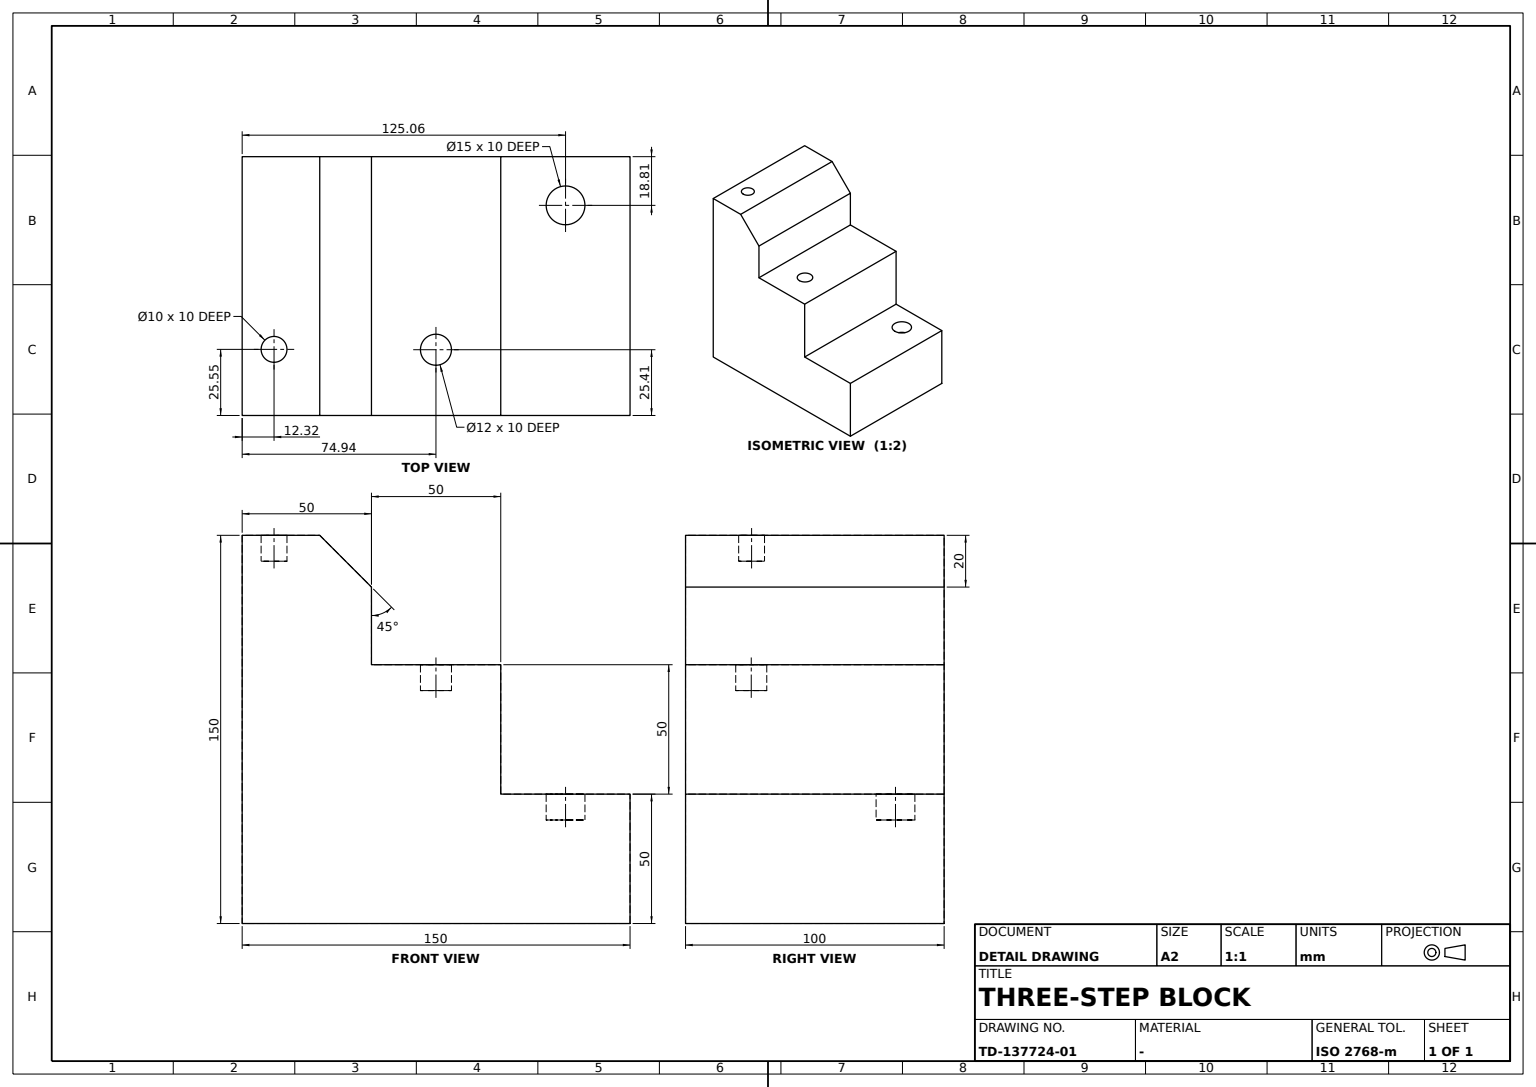
ISO-10303-21;
HEADER;
FILE_DESCRIPTION((''),'2;1');
FILE_NAME('','',(''),(''),'','','');
FILE_SCHEMA(('AUTOMOTIVE_DESIGN'));
ENDSEC;
DATA;
#1=APPLICATION_CONTEXT('');
#2=PRODUCT_CONTEXT('',#1,'mechanical');
#3=PRODUCT('','','',(#2));
#4=PRODUCT_DEFINITION_FORMATION('','',#3);
#5=PRODUCT_DEFINITION_CONTEXT('',#1,'design');
#6=PRODUCT_DEFINITION('','',#4,#5);
#7=PRODUCT_DEFINITION_SHAPE('','',#6);
#8=(LENGTH_UNIT()NAMED_UNIT(*)SI_UNIT(.MILLI.,.METRE.));
#9=(NAMED_UNIT(*)PLANE_ANGLE_UNIT()SI_UNIT($,.RADIAN.));
#10=(NAMED_UNIT(*)SI_UNIT($,.STERADIAN.)SOLID_ANGLE_UNIT());
#11=UNCERTAINTY_MEASURE_WITH_UNIT(LENGTH_MEASURE(0.005),#8,'distance_accuracy_value','');
#12=(GEOMETRIC_REPRESENTATION_CONTEXT(3)GLOBAL_UNCERTAINTY_ASSIGNED_CONTEXT((#11))GLOBAL_UNIT_ASSIGNED_CONTEXT((#8,#9,#10))REPRESENTATION_CONTEXT('',''));
#13=CARTESIAN_POINT('',(-50.,-75.,75.));
#14=VERTEX_POINT('',#13);
#15=CARTESIAN_POINT('',(50.,-75.,75.));
#16=VERTEX_POINT('',#15);
#17=CARTESIAN_POINT('',(0.,-75.,75.));
#18=DIRECTION('',(1.,0.,0.));
#19=VECTOR('',#18,1000.);
#20=LINE('',#17,#19);
#21=EDGE_CURVE('',#14,#16,#20,.T.);
#22=ORIENTED_EDGE('',*,*,#21,.F.);
#23=CARTESIAN_POINT('',(-50.,-75.,-75.));
#24=VERTEX_POINT('',#23);
#25=CARTESIAN_POINT('',(-50.,-75.,0.));
#26=DIRECTION('',(0.,0.,-1.));
#27=VECTOR('',#26,1000.);
#28=LINE('',#25,#27);
#29=EDGE_CURVE('',#14,#24,#28,.T.);
#30=ORIENTED_EDGE('',*,*,#29,.T.);
#31=CARTESIAN_POINT('',(50.,-75.,-75.));
#32=VERTEX_POINT('',#31);
#33=CARTESIAN_POINT('',(0.,-75.,-75.));
#34=LINE('',#33,#19);
#35=EDGE_CURVE('',#24,#32,#34,.T.);
#36=ORIENTED_EDGE('',*,*,#35,.T.);
#37=CARTESIAN_POINT('',(50.,-75.,0.));
#38=LINE('',#37,#27);
#39=EDGE_CURVE('',#16,#32,#38,.T.);
#40=ORIENTED_EDGE('',*,*,#39,.F.);
#41=EDGE_LOOP('',(#22,#30,#36,#40));
#42=FACE_BOUND('',#41,.T.);
#43=DIRECTION('',(0.,-1.,0.));
#44=AXIS2_PLACEMENT_3D('',#17,#43,#26);
#45=PLANE('',#44);
#46=ADVANCED_FACE('',(#42),#45,.T.);
#47=CARTESIAN_POINT('',(-38.687384,50.059444,-35.));
#48=VERTEX_POINT('',#47);
#49=CARTESIAN_POINT('',(-31.187384,50.059444,-35.));
#50=DIRECTION('',(-1.,0.,0.));
#51=AXIS2_PLACEMENT_3D('',#49,#26,#50);
#52=CIRCLE('',#51,7.5);
#53=EDGE_CURVE('',#48,#48,#52,.T.);
#54=ORIENTED_EDGE('',*,*,#53,.T.);
#55=EDGE_LOOP('',(#54));
#56=FACE_BOUND('',#55,.T.);
#57=CARTESIAN_POINT('',(-23.687384,50.059444,-25.));
#58=VERTEX_POINT('',#57);
#59=CARTESIAN_POINT('',(-31.187384,50.059444,-25.));
#60=DIRECTION('',(0.,0.,1.));
#61=AXIS2_PLACEMENT_3D('',#59,#60,#18);
#62=CIRCLE('',#61,7.5);
#63=EDGE_CURVE('',#58,#58,#62,.T.);
#64=ORIENTED_EDGE('',*,*,#63,.T.);
#65=EDGE_LOOP('',(#64));
#66=FACE_BOUND('',#65,.T.);
#67=CARTESIAN_POINT('',(-31.187384,50.059444,-25.1));
#68=AXIS2_PLACEMENT_3D('',#67,#26,#18);
#69=CYLINDRICAL_SURFACE('',#68,7.5);
#70=ADVANCED_FACE('',(#56,#66),#69,.F.);
#71=CARTESIAN_POINT('',(19.454487,-62.675179,65.));
#72=VERTEX_POINT('',#71);
#73=CARTESIAN_POINT('',(24.454487,-62.675179,65.));
#74=AXIS2_PLACEMENT_3D('',#73,#26,#50);
#75=CIRCLE('',#74,5.);
#76=EDGE_CURVE('',#72,#72,#75,.T.);
#77=ORIENTED_EDGE('',*,*,#76,.F.);
#78=EDGE_LOOP('',(#77));
#79=FACE_BOUND('',#78,.T.);
#80=AXIS2_PLACEMENT_3D('',#73,#26,#18);
#81=PLANE('',#80);
#82=ADVANCED_FACE('',(#79),#81,.F.);
#83=ORIENTED_EDGE('',*,*,#53,.F.);
#84=EDGE_LOOP('',(#83));
#85=FACE_BOUND('',#84,.T.);
#86=AXIS2_PLACEMENT_3D('',#49,#26,#18);
#87=PLANE('',#86);
#88=ADVANCED_FACE('',(#85),#87,.F.);
#89=CARTESIAN_POINT('',(-50.,25.,25.));
#90=VERTEX_POINT('',#89);
#91=CARTESIAN_POINT('',(50.,25.,25.));
#92=VERTEX_POINT('',#91);
#93=CARTESIAN_POINT('',(0.,25.,25.));
#94=LINE('',#93,#19);
#95=EDGE_CURVE('',#90,#92,#94,.T.);
#96=ORIENTED_EDGE('',*,*,#95,.F.);
#97=CARTESIAN_POINT('',(-50.,-25.,25.));
#98=VERTEX_POINT('',#97);
#99=CARTESIAN_POINT('',(-50.,0.,25.));
#100=VECTOR('',#43,1000.);
#101=LINE('',#99,#100);
#102=EDGE_CURVE('',#90,#98,#101,.T.);
#103=ORIENTED_EDGE('',*,*,#102,.T.);
#104=CARTESIAN_POINT('',(50.,-25.,25.));
#105=VERTEX_POINT('',#104);
#106=CARTESIAN_POINT('',(0.,-25.,25.));
#107=LINE('',#106,#19);
#108=EDGE_CURVE('',#98,#105,#107,.T.);
#109=ORIENTED_EDGE('',*,*,#108,.T.);
#110=CARTESIAN_POINT('',(50.,0.,25.));
#111=LINE('',#110,#100);
#112=EDGE_CURVE('',#92,#105,#111,.T.);
#113=ORIENTED_EDGE('',*,*,#112,.F.);
#114=EDGE_LOOP('',(#96,#103,#109,#113));
#115=FACE_BOUND('',#114,.T.);
#116=CARTESIAN_POINT('',(30.590931,-0.059691,25.));
#117=VERTEX_POINT('',#116);
#118=CARTESIAN_POINT('',(24.590931,-0.059691,25.));
#119=AXIS2_PLACEMENT_3D('',#118,#60,#18);
#120=CIRCLE('',#119,6.);
#121=EDGE_CURVE('',#117,#117,#120,.T.);
#122=ORIENTED_EDGE('',*,*,#121,.F.);
#123=EDGE_LOOP('',(#122));
#124=FACE_BOUND('',#123,.T.);
#125=AXIS2_PLACEMENT_3D('',#93,#60,#43);
#126=PLANE('',#125);
#127=ADVANCED_FACE('',(#115,#124),#126,.T.);
#128=CARTESIAN_POINT('',(-50.,25.,-25.));
#129=VERTEX_POINT('',#128);
#130=CARTESIAN_POINT('',(-50.,25.,0.));
#131=VECTOR('',#60,1000.);
#132=LINE('',#130,#131);
#133=EDGE_CURVE('',#129,#90,#132,.T.);
#134=ORIENTED_EDGE('',*,*,#133,.T.);
#135=ORIENTED_EDGE('',*,*,#95,.T.);
#136=CARTESIAN_POINT('',(50.,25.,-25.));
#137=VERTEX_POINT('',#136);
#138=CARTESIAN_POINT('',(50.,25.,0.));
#139=LINE('',#138,#131);
#140=EDGE_CURVE('',#137,#92,#139,.T.);
#141=ORIENTED_EDGE('',*,*,#140,.F.);
#142=CARTESIAN_POINT('',(0.,25.,-25.));
#143=LINE('',#142,#19);
#144=EDGE_CURVE('',#129,#137,#143,.T.);
#145=ORIENTED_EDGE('',*,*,#144,.F.);
#146=EDGE_LOOP('',(#134,#135,#141,#145));
#147=FACE_BOUND('',#146,.T.);
#148=DIRECTION('',(0.,1.,0.));
#149=AXIS2_PLACEMENT_3D('',#142,#148,#60);
#150=PLANE('',#149);
#151=ADVANCED_FACE('',(#147),#150,.T.);
#152=CARTESIAN_POINT('',(18.590931,-0.059691,15.));
#153=VERTEX_POINT('',#152);
#154=CARTESIAN_POINT('',(24.590931,-0.059691,15.));
#155=AXIS2_PLACEMENT_3D('',#154,#26,#50);
#156=CIRCLE('',#155,6.);
#157=EDGE_CURVE('',#153,#153,#156,.T.);
#158=ORIENTED_EDGE('',*,*,#157,.F.);
#159=EDGE_LOOP('',(#158));
#160=FACE_BOUND('',#159,.T.);
#161=AXIS2_PLACEMENT_3D('',#154,#26,#18);
#162=PLANE('',#161);
#163=ADVANCED_FACE('',(#160),#162,.F.);
#164=ORIENTED_EDGE('',*,*,#102,.F.);
#165=ORIENTED_EDGE('',*,*,#133,.F.);
#166=CARTESIAN_POINT('',(-50.,75.,-25.));
#167=VERTEX_POINT('',#166);
#168=CARTESIAN_POINT('',(-50.,0.,-25.));
#169=LINE('',#168,#100);
#170=EDGE_CURVE('',#167,#129,#169,.T.);
#171=ORIENTED_EDGE('',*,*,#170,.F.);
#172=CARTESIAN_POINT('',(-50.,75.,-75.));
#173=VERTEX_POINT('',#172);
#174=CARTESIAN_POINT('',(-50.,75.,0.));
#175=LINE('',#174,#131);
#176=EDGE_CURVE('',#173,#167,#175,.T.);
#177=ORIENTED_EDGE('',*,*,#176,.F.);
#178=CARTESIAN_POINT('',(-50.,0.,-75.));
#179=VECTOR('',#148,1000.);
#180=LINE('',#178,#179);
#181=EDGE_CURVE('',#24,#173,#180,.T.);
#182=ORIENTED_EDGE('',*,*,#181,.F.);
#183=ORIENTED_EDGE('',*,*,#29,.F.);
#184=CARTESIAN_POINT('',(-50.,-45.,75.));
#185=VERTEX_POINT('',#184);
#186=CARTESIAN_POINT('',(-50.,0.,75.));
#187=LINE('',#186,#100);
#188=EDGE_CURVE('',#185,#14,#187,.T.);
#189=ORIENTED_EDGE('',*,*,#188,.F.);
#190=CARTESIAN_POINT('',(-50.,-25.,55.));
#191=VERTEX_POINT('',#190);
#192=CARTESIAN_POINT('',(-50.,15.,15.));
#193=DIRECTION('',(0.,0.707106781,-0.707106781));
#194=VECTOR('',#193,1000.);
#195=LINE('',#192,#194);
#196=EDGE_CURVE('',#185,#191,#195,.T.);
#197=ORIENTED_EDGE('',*,*,#196,.T.);
#198=CARTESIAN_POINT('',(-50.,-25.,0.));
#199=LINE('',#198,#131);
#200=EDGE_CURVE('',#98,#191,#199,.T.);
#201=ORIENTED_EDGE('',*,*,#200,.F.);
#202=EDGE_LOOP('',(#164,#165,#171,#177,#182,#183,#189,#197,#201));
#203=FACE_BOUND('',#202,.T.);
#204=CARTESIAN_POINT('',(-50.,0.,0.));
#205=AXIS2_PLACEMENT_3D('',#204,#18,#148);
#206=PLANE('',#205);
#207=ADVANCED_FACE('',(#203),#206,.F.);
#208=CARTESIAN_POINT('',(50.,75.,-25.));
#209=VERTEX_POINT('',#208);
#210=CARTESIAN_POINT('',(0.,75.,-25.));
#211=LINE('',#210,#19);
#212=EDGE_CURVE('',#167,#209,#211,.T.);
#213=ORIENTED_EDGE('',*,*,#212,.T.);
#214=CARTESIAN_POINT('',(50.,75.,-75.));
#215=VERTEX_POINT('',#214);
#216=CARTESIAN_POINT('',(50.,75.,0.));
#217=LINE('',#216,#131);
#218=EDGE_CURVE('',#215,#209,#217,.T.);
#219=ORIENTED_EDGE('',*,*,#218,.F.);
#220=CARTESIAN_POINT('',(0.,75.,-75.));
#221=LINE('',#220,#19);
#222=EDGE_CURVE('',#173,#215,#221,.T.);
#223=ORIENTED_EDGE('',*,*,#222,.F.);
#224=ORIENTED_EDGE('',*,*,#176,.T.);
#225=EDGE_LOOP('',(#213,#219,#223,#224));
#226=FACE_BOUND('',#225,.T.);
#227=AXIS2_PLACEMENT_3D('',#220,#148,#60);
#228=PLANE('',#227);
#229=ADVANCED_FACE('',(#226),#228,.T.);
#230=CARTESIAN_POINT('',(29.454487,-62.675179,75.));
#231=VERTEX_POINT('',#230);
#232=CARTESIAN_POINT('',(24.454487,-62.675179,75.));
#233=AXIS2_PLACEMENT_3D('',#232,#60,#18);
#234=CIRCLE('',#233,5.);
#235=EDGE_CURVE('',#231,#231,#234,.T.);
#236=ORIENTED_EDGE('',*,*,#235,.T.);
#237=EDGE_LOOP('',(#236));
#238=FACE_BOUND('',#237,.T.);
#239=ORIENTED_EDGE('',*,*,#76,.T.);
#240=EDGE_LOOP('',(#239));
#241=FACE_BOUND('',#240,.T.);
#242=CARTESIAN_POINT('',(24.454487,-62.675179,74.9));
#243=AXIS2_PLACEMENT_3D('',#242,#26,#18);
#244=CYLINDRICAL_SURFACE('',#243,5.);
#245=ADVANCED_FACE('',(#238,#241),#244,.F.);
#246=CARTESIAN_POINT('',(50.,-45.,75.));
#247=VERTEX_POINT('',#246);
#248=CARTESIAN_POINT('',(50.,0.,75.));
#249=LINE('',#248,#100);
#250=EDGE_CURVE('',#247,#16,#249,.T.);
#251=ORIENTED_EDGE('',*,*,#250,.F.);
#252=CARTESIAN_POINT('',(70.,-45.,75.));
#253=VECTOR('',#50,1000.);
#254=LINE('',#252,#253);
#255=EDGE_CURVE('',#247,#185,#254,.T.);
#256=ORIENTED_EDGE('',*,*,#255,.T.);
#257=ORIENTED_EDGE('',*,*,#188,.T.);
#258=ORIENTED_EDGE('',*,*,#21,.T.);
#259=EDGE_LOOP('',(#251,#256,#257,#258));
#260=FACE_BOUND('',#259,.T.);
#261=ORIENTED_EDGE('',*,*,#235,.F.);
#262=EDGE_LOOP('',(#261));
#263=FACE_BOUND('',#262,.T.);
#264=CARTESIAN_POINT('',(0.,-25.,75.));
#265=AXIS2_PLACEMENT_3D('',#264,#60,#43);
#266=PLANE('',#265);
#267=ADVANCED_FACE('',(#260,#263),#266,.T.);
#268=CARTESIAN_POINT('',(50.,-25.,55.));
#269=VERTEX_POINT('',#268);
#270=CARTESIAN_POINT('',(0.,-25.,55.));
#271=LINE('',#270,#253);
#272=EDGE_CURVE('',#269,#191,#271,.T.);
#273=ORIENTED_EDGE('',*,*,#272,.T.);
#274=ORIENTED_EDGE('',*,*,#196,.F.);
#275=ORIENTED_EDGE('',*,*,#255,.F.);
#276=CARTESIAN_POINT('',(50.,15.,15.));
#277=LINE('',#276,#194);
#278=EDGE_CURVE('',#247,#269,#277,.T.);
#279=ORIENTED_EDGE('',*,*,#278,.T.);
#280=EDGE_LOOP('',(#273,#274,#275,#279));
#281=FACE_BOUND('',#280,.T.);
#282=DIRECTION('',(0.,-0.707106781,-0.707106781));
#283=AXIS2_PLACEMENT_3D('',#252,#282,#50);
#284=PLANE('',#283);
#285=ADVANCED_FACE('',(#281),#284,.F.);
#286=CARTESIAN_POINT('',(50.,0.,-75.));
#287=LINE('',#286,#179);
#288=EDGE_CURVE('',#32,#215,#287,.T.);
#289=ORIENTED_EDGE('',*,*,#288,.F.);
#290=ORIENTED_EDGE('',*,*,#35,.F.);
#291=ORIENTED_EDGE('',*,*,#181,.T.);
#292=ORIENTED_EDGE('',*,*,#222,.T.);
#293=EDGE_LOOP('',(#289,#290,#291,#292));
#294=FACE_BOUND('',#293,.T.);
#295=AXIS2_PLACEMENT_3D('',#33,#26,#148);
#296=PLANE('',#295);
#297=ADVANCED_FACE('',(#294),#296,.T.);
#298=ORIENTED_EDGE('',*,*,#212,.F.);
#299=ORIENTED_EDGE('',*,*,#170,.T.);
#300=ORIENTED_EDGE('',*,*,#144,.T.);
#301=CARTESIAN_POINT('',(50.,0.,-25.));
#302=LINE('',#301,#100);
#303=EDGE_CURVE('',#209,#137,#302,.T.);
#304=ORIENTED_EDGE('',*,*,#303,.F.);
#305=EDGE_LOOP('',(#298,#299,#300,#304));
#306=FACE_BOUND('',#305,.T.);
#307=ORIENTED_EDGE('',*,*,#63,.F.);
#308=EDGE_LOOP('',(#307));
#309=FACE_BOUND('',#308,.T.);
#310=AXIS2_PLACEMENT_3D('',#210,#60,#43);
#311=PLANE('',#310);
#312=ADVANCED_FACE('',(#306,#309),#311,.T.);
#313=ORIENTED_EDGE('',*,*,#112,.T.);
#314=CARTESIAN_POINT('',(50.,-25.,0.));
#315=LINE('',#314,#131);
#316=EDGE_CURVE('',#105,#269,#315,.T.);
#317=ORIENTED_EDGE('',*,*,#316,.T.);
#318=ORIENTED_EDGE('',*,*,#278,.F.);
#319=ORIENTED_EDGE('',*,*,#250,.T.);
#320=ORIENTED_EDGE('',*,*,#39,.T.);
#321=ORIENTED_EDGE('',*,*,#288,.T.);
#322=ORIENTED_EDGE('',*,*,#218,.T.);
#323=ORIENTED_EDGE('',*,*,#303,.T.);
#324=ORIENTED_EDGE('',*,*,#140,.T.);
#325=EDGE_LOOP('',(#313,#317,#318,#319,#320,#321,#322,#323,#324));
#326=FACE_BOUND('',#325,.T.);
#327=CARTESIAN_POINT('',(50.,0.,0.));
#328=AXIS2_PLACEMENT_3D('',#327,#18,#148);
#329=PLANE('',#328);
#330=ADVANCED_FACE('',(#326),#329,.T.);
#331=ORIENTED_EDGE('',*,*,#272,.F.);
#332=ORIENTED_EDGE('',*,*,#316,.F.);
#333=ORIENTED_EDGE('',*,*,#108,.F.);
#334=ORIENTED_EDGE('',*,*,#200,.T.);
#335=EDGE_LOOP('',(#331,#332,#333,#334));
#336=FACE_BOUND('',#335,.T.);
#337=AXIS2_PLACEMENT_3D('',#106,#148,#60);
#338=PLANE('',#337);
#339=ADVANCED_FACE('',(#336),#338,.T.);
#340=ORIENTED_EDGE('',*,*,#121,.T.);
#341=EDGE_LOOP('',(#340));
#342=FACE_BOUND('',#341,.T.);
#343=ORIENTED_EDGE('',*,*,#157,.T.);
#344=EDGE_LOOP('',(#343));
#345=FACE_BOUND('',#344,.T.);
#346=CARTESIAN_POINT('',(24.590931,-0.059691,24.9));
#347=AXIS2_PLACEMENT_3D('',#346,#26,#18);
#348=CYLINDRICAL_SURFACE('',#347,6.);
#349=ADVANCED_FACE('',(#342,#345),#348,.F.);
#350=CLOSED_SHELL('',(#46,#70,#82,#88,#127,#151,#163,#207,#229,#245,#267,#285,#297,#312,#330,#339,#349));
#351=MANIFOLD_SOLID_BREP('',#350);
#352=ADVANCED_BREP_SHAPE_REPRESENTATION('',(#351),#12);
#353=SHAPE_DEFINITION_REPRESENTATION(#7,#352);
ENDSEC;
END-ISO-10303-21;
